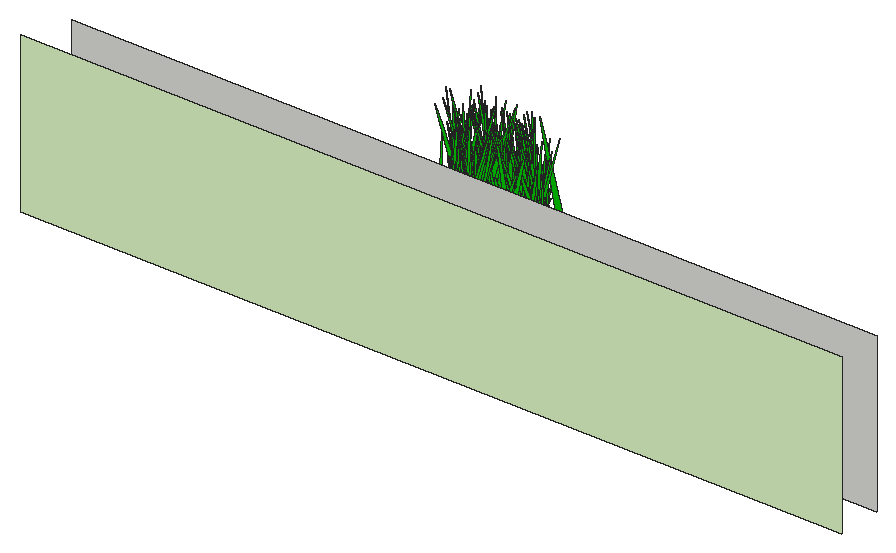
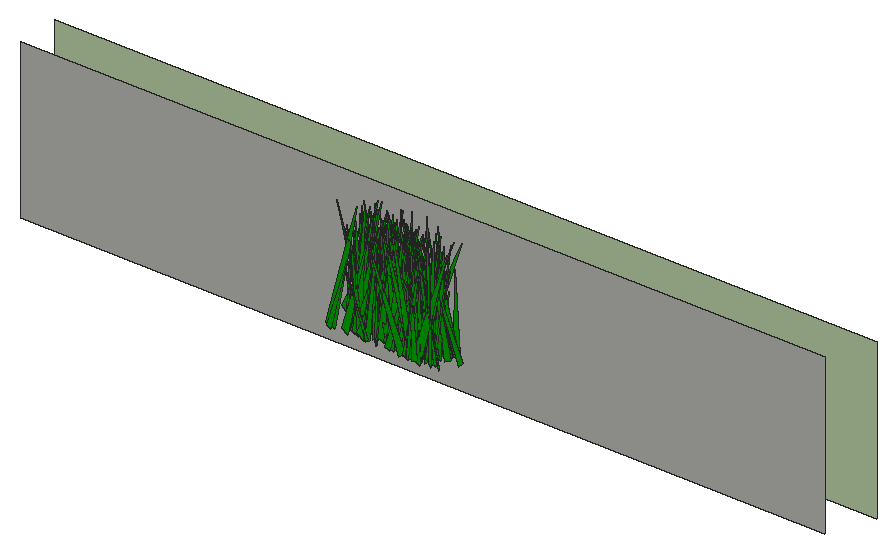
# SketchUp Ruby script. Lengths in inches.
U = 1.inch
M = Sketchup.active_model
def pt(a) = Geom::Point3d.new(a.map { |v| v * U })
def face(e, loops, mat)
  f = e.add_face(loops[0].map { |a| pt(a) })
  loops[1..].each { |l| e.add_face(l.map { |a| pt(a) }).erase! }
  f.material = f.back_material = mat if mat
  f
end
# faces: each face lists its corners as indices into pts; further lists are holes
def faces(e, pts, list, mat = nil) = list.each { |f| face(e, (f[0].is_a?(Array) ? f : [f]).map { |l| l.map { |i| pts[i] } }, mat) }
# xy, xz, yz: faces in a plane at the given z, y or x. An outline is a flat list of corners, or four numbers for a rectangle; further outlines are holes
def ring(l) = l.size == 4 ? [[l[0], l[1]], [l[2], l[1]], [l[2], l[3]], [l[0], l[3]]] : l.each_slice(2).to_a
def flat(e, list, mat, &to3) = list.each { |f| face(e, (f[0].is_a?(Array) ? f : [f]).map { |l| ring(l).map { |u, v| to3.(u, v) } }, mat) }
def xy(e, z, list, mat = nil) = flat(e, list, mat) { |x, y| [x, y, z] }
def xz(e, y, list, mat = nil) = flat(e, list, mat) { |x, z| [x, y, z] }
def yz(e, x, list, mat = nil) = flat(e, list, mat) { |y, z| [x, y, z] }
def lines(e, pts, list) = list.each { |a, b| e.add_line(pt(pts[a]), pt(pts[b])) }
# prism: a flat outline (further loops are holes) pulled along v
def prism(e, loops, v, mat = nil)
  f = face(e, loops, mat); d = Geom::Vector3d.new(v.map { |x| x * U })
  f.pushpull(f.normal.samedirection?(d) ? d.length : -d.length)
end
def box(e, o, s, mat = nil) = prism(e, [[o, [o[0] + s[0], o[1], o[2]], [o[0] + s[0], o[1] + s[1], o[2]], [o[0], o[1] + s[1], o[2]]]], [0, 0, s[2]], mat)
def at(x, y, z, deg = 0) = Geom::Transformation.translation(pt([x, y, z])) * Geom::Transformation.rotation(ORIGIN, Z_AXIS, deg.degrees)
def axes(o, x, y, z) = Geom::Transformation.new([*x, 0, *y, 0, *z, 0, *pt(o).to_a, 1])
def part(name) = M.definitions.add(name)
# library, detail: a bought-in or finely detailed component or shape, given as its bounding box
def library(name, o, s) = part(name).tap { |d| box(d.entities, o, s) }
def detail(e, o, s) = box(e.add_group.entities, o, s)
def put(e, d, t, mat = nil) = e.add_instance(d, t).tap { |i| i.material = mat if mat }
def group(e, t, mat = nil) = e.add_group.tap { |g| g.transformation = t; g.material = mat if mat }.entities
root = M.entities
M.materials.add("[Color F01]1").color = [229, 255, 204]
M.materials.add("[Color G06]").color = [0, 204, 0]
c1 = part("fur_instance\#9")
p = [[0.8125,0,1.79],[0.67,-0.02,1.48],[0,-0.11,0],[0,0.11,0]]
faces(c1.entities,p,[[0,1,2,3]])
xz(root,2.125,[[0,-6,121.48,17.375]],"[Color F01]1")
xz(root,8.54,[[2.44,-6,121.48,17.375]])
put(root,c1,axes([51.91,18.98,4.28],[-5.43727,-0.1309,1.77708],[-1.14633,0.75939,-1.4087],[0.99043,0.16028,8.12542]),"[Color G06]")
put(root,c1,axes([50.8,16.22,4.28],[1.59166,0.55171,0.19188],[3.87124,-0.22097,1.25545],[-0.82664,0.02745,6.24887]),"[Color G06]")
put(root,c1,axes([50.67,17.92,4.28],[2.66118,-0.06056,1.5398],[-0.73116,-0.37487,1.12897],[-0.84584,0.1335,3.86858]),"[Color G06]")
put(root,c1,axes([52.11,18.91,4.28],[-4.41289,-0.15737,0.71019],[-0.90608,0.58635,2.34948],[0.82368,-0.19812,6.38937]),"[Color G06]")
put(root,c1,axes([50.03,20.49,4.28],[3.21331,-0.02062,0.29283],[-0.07963,-0.42686,-1.50113],[-0.23219,-0.13898,4.56724]),"[Color G06]")
put(root,c1,axes([53.29,20.63,4.28],[-0.32371,-0.80099,1.32155],[-5.37319,-0.00581,-3.34481],[-2.21483,0.13118,7.92139]),"[Color G06]")
put(root,c1,axes([50.27,17.08,4.28],[-0.50903,0.54466,0.68853],[3.72815,0.08745,-1.79039],[1.2527,-0.03895,5.60818]),"[Color G06]")
put(root,c1,axes([48.65,18.15,4.28],[3.59181,0.48472,0.30488],[3.26872,-0.45529,-2.86735],[1.19994,-0.21067,6.89826]),"[Color G06]")
put(root,c1,axes([51.4,20.41,4.28],[-3.58351,-0.18608,3.16742],[-1.99042,0.52471,-1.48906],[1.51995,0.24842,5.51771]),"[Color G06]")
put(root,c1,axes([53.17,19.5,4.28],[-2.59947,0.59847,0.19892],[4.24015,0.35436,1.30133],[-0.67711,-0.07856,7.38549]),"[Color G06]")
put(root,c1,axes([51.89,18.54,4.28],[1.47697,-0.74428,0.0462],[-5.2567,-0.20361,-1.42243],[-0.9254,-0.0313,8.15384]),"[Color G06]")
put(root,c1,axes([52.12,20.3,4.28],[-2.67483,-0.2008,0.45513],[-1.28725,0.36186,1.44134],[0.7137,-0.09992,4.30538]),"[Color G06]")
put(root,c1,axes([50.39,18.45,4.28],[2.14413,0.52359,3.01188],[4.23289,-0.22537,-2.23054],[0.49195,-0.34289,6.06514]),"[Color G06]")
put(root,c1,axes([51.79,19.5625,4.28],[-3.356,-0.37288,1.10105],[-2.37095,0.46935,2.11661],[1.43931,-0.09628,6.05393]),"[Color G06]")
put(root,c1,axes([52.37,16.84,4.28],[1.56901,0.37265,0.88402],[2.38955,-0.23286,1.80258],[-1.33471,0.02117,4.2664]),"[Color G06]")
put(root,c1,axes([51.46,20.07,4.28],[-1.02275,-0.37605,1.39838],[-2.66112,0.17575,1.08178],[1.03265,0.08046,4.17267]),"[Color G06]")
put(root,c1,axes([52.05,16.48,4.28],[3.73089,0.48313,0.10401],[2.99318,-0.45646,3.73766],[-1.74634,0.24981,6.62847]),"[Color G06]")
put(root,c1,axes([50.84,17.53,4.28],[1.44178,-0.46037,0.51457],[-3.24906,-0.18502,1.31972],[0.67931,0.09216,5.21997]),"[Color G06]")
put(root,c1,axes([51.3,20.03,4.28],[4.4532,-0.59952,0.68935],[-4.15792,-0.61906,-1.84914],[-1.18686,-0.08069,9.06462]),"[Color G06]")
put(root,c1,axes([53.47,17.11,4.28],[-4.54302,0.12366,0.66916],[0.73291,0.61451,-1.93068],[0.67062,0.16614,6.64316]),"[Color G06]")
put(root,c1,axes([50.8,17.34,4.28],[2.63054,0.38998,0.98746],[2.84635,-0.33642,-1.67464],[0.3952,-0.17281,5.48849]),"[Color G06]")
put(root,c1,axes([55.2,16.72,4.28],[-0.3206,-0.72645,3.92377],[-5.03987,-0.15016,-4.11338],[-2.93792,0.33686,6.62813]),"[Color G06]")
put(root,c1,axes([51.51,19.54,4.28],[5.2193,-0.28703,1.37107],[-1.85383,-0.73035,-1.80051],[-1.28134,-0.11251,8.18977]),"[Color G06]")
put(root,c1,axes([53.89,18,4.28],[-1.41177,0.69633,0.61405],[4.93285,0.18273,1.52968],[-0.87839,-0.093,7.60345]),"[Color G06]")
put(root,c1,axes([51.71,18.59,4.28],[3.12751,-0.10134,1.06954],[-0.89259,-0.42768,1.17512],[-0.4935,0.13131,4.65273]),"[Color G06]")
put(root,c1,axes([51.93,19.64,4.28],[-0.34521,0.71417,0.85118],[5.04938,0.06277,-1.47542],[1.02858,-0.06844,7.52863]),"[Color G06]")
put(root,c1,axes([51.91,17.48,4.28],[5.4788,-0.35623,0.70633],[-2.08372,-0.6944,-4.12755],[-1.55165,-0.32532,8.03693]),"[Color G06]")
put(root,c1,axes([52.09,16.08,4.28],[-3.28322,0.56965,2.82631],[3.90028,0.52294,-1.98729],[2.24771,-0.07533,7.57675]),"[Color G06]")
put(root,c1,axes([53.39,18.09,4.28],[1.26443,0.71457,1.55863],[5.10243,-0.20135,1.35812],[-1.1454,-0.10814,7.77067]),"[Color G06]")
put(root,c1,axes([53.06,20.23,4.28],[2.01762,0.51142,0.00605],[3.4996,-0.26866,1.86814],[-1.09703,0.08354,5.97064]),"[Color G06]")
put(root,c1,axes([53.86,16.875,4.28],[-2.81215,0.18439,1.24159],[1.54852,0.36006,1.69194],[0.2015,-0.19378,4.32525]),"[Color G06]")
put(root,c1,axes([52.39,19.39,4.28],[5.28794,0.45044,0.30203],[2.73932,-0.65163,4.5076],[-1.7237,0.34626,8.09011]),"[Color G06]")
put(root,c1,axes([53.04,20.05,4.28],[-1.73279,-0.44896,0.00822],[-3.13171,0.23524,1.26378],[0.74712,-0.05522,5.31643]),"[Color G06]")
put(root,c1,axes([56.03,17.67,4.28],[-4.70247,0.53813,0.21183],[3.67167,0.61341,3.06077],[-1.19634,-0.23262,8.56112]),"[Color G06]")
put(root,c1,axes([52.2,17.94,4.28],[-0.36312,-0.73049,0.03256],[-5.06328,0.04972,2.01132],[1.34399,-0.01005,7.58611]),"[Color G06]")
put(root,c1,axes([53.14,19.85,4.28],[2.57444,0.09347,1.0726],[0.37331,-0.35287,1.53085],[-0.90827,0.11989,3.66944]),"[Color G06]")
put(root,c1,axes([51.55,17.57,4.28],[4.954,0.01736,0.01736],[0.11791,-0.67006,1.80205],[-0.04155,0.16804,7.18388]),"[Color G06]")
put(root,c1,axes([53.58,18.73,4.28],[-2.17917,0.34186,0.81991],[2.32851,0.31287,-1.1613],[0.9429,0.01744,4.76276]),"[Color G06]")
put(root,c1,axes([51.83,17.94,4.28],[2.92636,-0.57671,1.37096],[-4.19516,-0.37292,1.98178],[0.58866,0.20931,7.30812]),"[Color G06]")
put(root,c1,axes([53.86,19.83,4.28],[0.93646,-0.35885,0.31759],[-2.46765,-0.13365,-1.09467],[-0.76036,-0.0082,3.94375]),"[Color G06]")
put(root,c1,axes([54.26,15.89,4.28],[-3.0515,0.17993,1.51687],[1.52303,0.42177,1.09675],[0.61266,-0.15232,4.82866]),"[Color G06]")
put(root,c1,axes([53.98,16.67,4.28],[-2.96455,0.01566,1.45683],[-0.26452,0.40381,-1.70114],[0.94487,0.16219,4.09459]),"[Color G06]")
put(root,c1,axes([53.41,17.24,4.28],[-2.20301,-0.3923,0.30621],[-2.46722,0.28556,2.37694],[1.36733,-0.11681,4.78234]),"[Color G06]")
put(root,c1,axes([52.2,19.61,4.28],[2.68315,-0.56541,1.54609],[-4.15271,-0.33867,1.87057],[0.51547,0.21471,7.02186]),"[Color G06]")
put(root,c1,axes([54.77,17.11,4.28],[-3.65389,0.39957,2.10603],[3.14363,0.50252,1.23084],[0.56016,-0.21377,6.82994]),"[Color G06]")
put(root,c1,axes([53.4375,20.73,4.28],[-1.09405,-0.45265,0.62127],[-3.12842,0.1626,1.30294],[0.96057,0.01401,4.95104]),"[Color G06]")
put(root,c1,axes([54.01,16.18,4.28],[-3.79355,0.174,2.16516],[1.06017,0.56495,-1.06638],[1.59116,0.03843,5.87255]),"[Color G06]")
put(root,c1,axes([55.3,20.36,4.28],[0.09839,-0.76811,0.41834],[-5.27928,-0.02442,-2.37631],[-1.59654,0.0334,7.88352]),"[Color G06]")
put(root,c1,axes([54.09,17.07,4.28],[-2.01588,0.37847,0.07105],[2.59123,0.27075,-1.45532],[0.80893,0.07587,4.83886]),"[Color G06]")
put(root,c1,axes([54.8125,20.64,4.28],[1.79807,-0.46544,1.83512],[-3.12533,-0.29835,-1.85243],[-1.69731,0.0563,5.35503]),"[Color G06]")
put(root,c1,axes([55.7,20.13,4.28],[-4.8184,-0.1577,1.09211],[-1.30772,0.63828,-2.30012],[0.32064,0.23332,7.03046]),"[Color G06]")
put(root,c1,axes([54.84,20.6,4.28],[-5.6317,-0.0853,2.59145],[-0.41065,0.81772,1.09845],[1.79219,-0.08067,8.39493]),"[Color G06]")
put(root,c1,axes([56.25,17.3,4.28],[-0.91344,0.56581,1.68311],[3.78284,0.03966,3.05415],[-1.84997,-0.19827,5.41411]),"[Color G06]")
put(root,c1,axes([53.04,16.04,4.28],[5.03717,-0.2836,0.52782],[-1.87621,-0.68318,-2.17154],[-0.86065,-0.1705,7.82309]),"[Color G06]")
put(root,c1,axes([54.01,19.33,4.28],[-2.92682,0.64675,1.27318],[4.37587,0.4246,-2.30737],[1.75749,0.01987,7.86524]),"[Color G06]")
put(root,c1,axes([54.18,16.9,4.28],[-4.87066,0.13601,5.05112],[2.2494,0.73928,2.55826],[2.70436,-0.36995,6.96939]),"[Color G06]")
put(root,c1,axes([54.86,18.23,4.28],[3.21289,-0.35741,2.23312],[-2.45895,-0.49264,-1.15504],[-1.65999,0.03798,6.03315]),"[Color G06]")
put(root,c1,axes([55.24,17.59,4.28],[-4.44876,-0.50622,0.53471],[-3.31452,0.59382,2.98091],[1.52335,-0.18632,8.04742]),"[Color G06]")
put(root,c1,axes([56.57,19.68,4.28],[-4.95682,0.3204,1.78327],[2.56581,0.65591,2.3934],[0.34564,-0.27427,7.80688]),"[Color G06]")
put(root,c1,axes([54.06,18.78,4.28],[5.71057,0.15561,1.7452],[0.49355,-0.73778,3.94943],[-1.53791,0.34103,7.74774]),"[Color G06]")
put(root,c1,axes([56.01,16.83,4.28],[-3.14332,-0.06886,0.79043],[-0.6143,0.42769,-1.17654],[0.38237,0.12102,4.6077]),"[Color G06]")
put(root,c1,axes([54.67,19.4,4.28],[4.9091,-0.22213,1.7695],[-1.06395,-0.66635,-3.01583],[-1.67549,-0.22769,7.09963]),"[Color G06]")
put(root,c1,axes([53.87,17.86,4.28],[0.98414,-0.63505,2.16198],[-4.67123,-0.0845,1.89848],[1.00608,0.22887,6.6998]),"[Color G06]")
put(root,c1,axes([57.23,16.93,4.28],[-0.71373,0.56558,2.16635],[3.82854,-0.01056,3.13415],[-1.97327,-0.22505,5.29731]),"[Color G06]")
put(root,c1,axes([53.07,18.01,4.28],[4.3109,0.57571,0.91743],[4.15372,-0.57961,-1.81566],[0.41065,-0.18096,8.7344]),"[Color G06]")
put(root,c1,axes([56.8125,16.01,4.28],[-5.14763,-0.11078,0.62818],[-0.69238,0.70606,1.62962],[0.57303,-0.14201,7.6121]),"[Color G06]")
put(root,c1,axes([54.51,19.01,4.28],[4.6637,0.04467,1.96815],[0.56634,-0.66207,-1.27146],[-1.23126,-0.13533,6.87]),"[Color G06]")
put(root,c1,axes([54.84,16.01,4.28],[-2.53601,-0.44544,1.887],[-2.94328,0.39463,1.86527],[1.77059,0.018,5.8034]),"[Color G06]")
put(root,c1,axes([55.8,19.72,4.28],[-4.87145,-0.24567,2.22206],[-1.45468,0.70359,1.8125],[1.78837,-0.0969,7.52712]),"[Color G06]")
put(root,c1,axes([54.28,16.97,4.28],[3.75989,-0.18432,0.02514],[-1.26237,-0.50274,-1.6992],[-0.39228,-0.14882,5.70906]),"[Color G06]")
put(root,c1,axes([54.05,20.52,4.28],[3.78708,-0.61294,1.46517],[-4.50316,-0.51295,1.34878],[0.0613,0.18561,8.56597]),"[Color G06]")
put(root,c1,axes([57.54,19.3,4.28],[-0.2302,-0.7663,3.67987],[-5.72631,-0.07844,-2.6766],[-1.86297,0.33579,7.77248]),"[Color G06]")
put(root,c1,axes([57.55,18.17,4.28],[-4.41754,0.41018,1.19465],[3.04744,0.59864,1.55983],[0.06736,-0.18307,7.77723]),"[Color G06]")
put(root,c1,axes([57.73,18.14,4.28],[-2.28217,0.3951,0.98803],[2.74251,0.25301,2.52763],[-0.97151,-0.21392,4.81436]),"[Color G06]")
put(root,c1,axes([54.64,16.04,4.28],[4.80796,0.27285,0.51449],[1.85051,-0.66078,1.62678],[-0.72295,0.1232,7.58565]),"[Color G06]")
put(root,c1,axes([55.62,18.85,4.28],[-2.56409,0.55267,1.28765],[3.73312,0.37715,-1.99047],[1.58564,0.00577,6.76845]),"[Color G06]")
put(root,c1,axes([57,16.68,4.28],[-2.39553,-0.28305,0.99137],[-2.13538,0.31619,-1.15524],[-0.02023,0.142,4.54836]),"[Color G06]")
put(root,c1,axes([56.44,18.59,4.28],[-3.57468,0.37857,0.89322],[2.5316,0.49942,-1.68408],[1.14822,0.07745,6.49389]),"[Color G06]")
put(root,c1,axes([56.22,19.31,4.28],[-3.25199,-0.42833,0.48071],[-2.81575,0.43795,2.27741],[1.26886,-0.12592,6.28583]),"[Color G06]")
put(root,c1,axes([56.7,18.07,4.28],[-5.02578,0.41451,1.36063],[2.66068,0.69831,-2.48577],[1.60806,0.14008,8.36541]),"[Color G06]")
put(root,c1,axes([55.55,18.9,4.28],[5.31584,-0.3496,1.58327],[-2.05145,-0.72768,-3.07238],[-1.78863,-0.20441,8.22934]),"[Color G06]")
put(root,c1,axes([55.73,17.21,4.28],[2.97516,0.3331,0.52522],[2.22924,-0.40884,1.57847],[-0.92733,0.08584,5.47962]),"[Color G06]")
put(root,c1,axes([54.18,16.14,4.28],[4.72016,-0.32932,0.82208],[-2.4235,-0.63512,1.85574],[0.08048,0.18904,7.66695]),"[Color G06]")
put(root,c1,axes([53.94,20.49,4.28],[2.61336,-0.7133,1.78302],[-5.079,-0.2958,3.03462],[1.33898,0.27014,8.03086]),"[Color G06]")
put(root,c1,axes([52.64,16.54,4.28],[3.88839,-0.66133,0.92114],[-4.20681,-0.42029,5.00392],[2.27473,0.35318,7.67952]),"[Color G06]")
put(root,c1,axes([57.01,18.27,4.28],[0.09928,0.6289,0.73743],[4.45999,-0.02615,1.22031],[-0.83184,-0.06513,6.63078]),"[Color G06]")
put(root,c1,axes([56.4,18.125,4.28],[-3.14788,-0.71939,1.72009],[-5.10547,0.46218,1.33437],[1.36872,0.06948,8.93334]),"[Color G06]")
put(root,c1,axes([57.7,20.47,4.28],[-1.20173,-0.48488,0.32642],[-3.34679,0.1517,-1.63607],[-0.96834,0.07743,5.24951]),"[Color G06]")
put(root,c1,axes([56.45,18.53,4.28],[-3.24455,0.24157,1.31211],[1.29837,0.44707,-2.28355],[1.44431,0.14078,5.00039]),"[Color G06]")
put(root,c1,axes([54.61,15.99,4.28],[3.56814,-0.46325,0.26466],[-3.29258,-0.48656,1.32268],[0.476,0.10693,7.16534]),"[Color G06]")
put(root,c1,axes([56.65,18.36,4.28],[4.28936,-0.1549,2.53842],[-0.25097,-0.59001,-3.18872],[-2.01387,-0.2564,5.80399]),"[Color G06]")
put(root,c1,axes([58.7,19.6,4.28],[-2.42071,-0.34779,0.35927],[-2.18179,0.26965,-2.85087],[-1.2321,0.2058,4.34246]),"[Color G06]")
put(root,c1,axes([55.77,16.59,4.28],[2.0153,0.3765,1.5154],[2.88365,-0.2601,-1.14271],[0.04918,-0.17695,4.90408]),"[Color G06]")
put(root,c1,axes([57.52,20.24,4.28],[0.89482,-0.73405,1.78711],[-5.23661,-0.15908,-1.64899],[-1.31072,0.13441,7.80815]),"[Color G06]")
put(root,c1,axes([57,18,4.28],[2.87944,0.06028,2.41609],[0.89575,-0.43448,-1.13929],[-1.41345,-0.15254,4.19998]),"[Color G06]")
put(root,c1,axes([55.72,18.04,4.28],[1.49486,-0.57441,0.15573],[-4.06287,-0.20289,1.14753],[0.68695,0.04998,6.44801]),"[Color G06]")
put(root,c1,axes([56.75,18.97,4.28],[-4.2817,-0.58541,2.60043],[-3.99315,0.6438,1.96254],[2.16944,0.0296,8.74461]),"[Color G06]")
put(root,c1,axes([59.28,18.55,4.28],[-6.16398,0.00446,0.29622],[-0.01792,0.83336,-2.2759],[0.19996,0.21231,8.92709]),"[Color G06]")
put(root,c1,axes([55.78,16.93,4.28],[0.20196,0.67568,1.34421],[4.7415,0.00758,-2.02915],[1.34367,-0.12832,6.95834]),"[Color G06]")
put(root,c1,axes([58.15,19.48,4.28],[-4.96916,-0.37311,0.63335],[-2.44496,0.67085,2.5494],[1.16665,-0.18332,8.0405]),"[Color G06]")
put(root,c1,axes([58.1,16.55,4.28],[-3.33094,0.10151,1.09293],[0.89973,0.45444,1.27666],[0.50511,-0.14009,4.93332]),"[Color G06]")
put(root,c1,axes([59.75,17.29,4.28],[-1.76106,0.73325,1.58639],[4.99783,0.16767,3.4903],[-1.94889,-0.23259,7.51719]),"[Color G06]")
put(root,c1,axes([55.82,17.77,4.28],[0.02607,0.52347,2.26385],[3.70064,0.08253,-2.2873],[1.64064,-0.19446,5.12328]),"[Color G06]")
put(root,c1,axes([56.61,16.125,4.28],[-1.26157,0.51868,2.58255],[3.837,0.2383,-1.31112],[1.44861,-0.1795,5.72193]),"[Color G06]")
put(root,c1,axes([57.54,17.97,4.28],[1.91115,0.38665,0.83998],[2.64993,-0.27777,1.2201],[-0.99089,0.00289,4.88298]),"[Color G06]")
put(root,c1,axes([57.68,18.73,4.28],[-3.11151,-0.45224,0.51795],[-3.0544,0.42745,1.88682],[1.14395,-0.08877,6.44672]),"[Color G06]")
put(root,c1,axes([55.51,16.04,4.28],[4.67702,0.23225,0.60128],[1.71295,-0.62979,-1.81715],[0.04177,-0.17849,7.19422]),"[Color G06]")
put(root,c1,axes([58.64,16.68,4.28],[-0.52684,0.57055,1.22282],[4.03527,0.04041,1.71746],[-1.06157,-0.12954,5.9216]),"[Color G06]")
put(root,c1,axes([59.4375,17.36,4.28],[-4.19523,-0.33988,0.94339],[-2.51196,0.55339,-2.04935],[-0.1711,0.20914,6.95587]),"[Color G06]")
put(root,c1,axes([56.38,15.94,4.28],[4.69206,-0.25919,1.77415],[-2.06215,-0.65357,1.21386],[-0.78195,0.16834,7.4445]),"[Color G06]")
put(root,c1,axes([55.08,17.45,4.28],[3.63127,0.64495,2.15055],[4.69378,-0.40661,-3.69554],[1.19603,-0.36239,7.97377]),"[Color G06]")
put(root,c1,axes([56.2,19.58,4.28],[0.70458,0.81412,1.97938],[5.8353,-0.05186,-2.18973],[1.33732,-0.20266,8.51186]),"[Color G06]")
put(root,c1,axes([56.64,19.93,4.28],[-0.72254,-0.69652,2.04973],[-4.94896,0.14983,1.95188],[1.52905,0.15581,7.28607]),"[Color G06]")
put(root,c1,axes([57.56,18.86,4.28],[2.95462,-0.61198,0.5839],[-4.26992,-0.41389,-1.56813],[-1.08657,-0.03764,7.75007]),"[Color G06]")
put(root,c1,axes([55.51,20.54,4.28],[3.63201,-0.5608,0.16417],[-3.79812,-0.47116,2.81005],[1.32659,0.18642,7.59589]),"[Color G06]")
put(root,c1,axes([57.04,18.49,4.28],[0.96081,-0.78066,1.91846],[-5.66561,-0.09902,1.70963],[0.94316,0.20046,8.31548]),"[Color G06]")
put(root,c1,axes([59.49,20.31,4.28],[-5.21835,0.0177,1.63396],[-0.14397,0.7214,-1.92453],[1.09115,0.17981,7.56041]),"[Color G06]")
put(root,c1,axes([60.48,17.36,4.28],[-1.76784,0.57266,1.28932],[3.92784,0.17988,2.85242],[-1.47686,-0.20709,6.0429]),"[Color G06]")
put(root,c1,axes([59.72,16.93,4.28],[-2.41599,0.39074,1.41292],[2.94773,0.30452,1.58494],[-0.23753,-0.19532,5.29768]),"[Color G06]")
put(root,c1,axes([59.74,19.23,4.28],[1.52959,0.68165,3.45387],[5.03204,-0.302,1.869],[-1.97854,-0.24111,7.42359]),"[Color G06]")
put(root,c1,axes([58.77,18.43,4.28],[-3.12089,-0.21213,1.44841],[-1.33071,0.4531,1.21818],[1.21756,-0.04852,5.04398]),"[Color G06]")
put(root,c1,axes([59.61,19.3,4.28],[-0.63491,0.58858,0.91286],[4.20465,0.07198,1.20142],[-0.71378,-0.09956,6.26518]),"[Color G06]")
put(root,c1,axes([62.25,18.44,4.28],[-3.78619,0.6952,0.26747],[4.53583,0.46669,4.07886],[-2.07688,-0.24814,8.42047]),"[Color G06]")
put(root,c1,axes([60.36,18.36,4.28],[-5.22329,0.32936,0.9818],[2.26179,0.73058,-1.27526],[0.94575,0.0718,8.47217]),"[Color G06]")
put(root,c1,axes([59.44,17.84,4.28],[-4.03787,-0.59657,0.40051],[-4.00136,0.54299,2.79815],[1.53731,-0.15362,8.33506]),"[Color G06]")
put(root,c1,axes([58.2,16.96,4.28],[2.92501,-0.11015,0.95],[-0.99431,-0.36461,1.98179],[-0.19851,0.20317,4.07157]),"[Color G06]")
put(root,c1,axes([59.71,18,4.28],[-5.12636,-0.18079,2.7137],[-0.9747,0.7522,1.64386],[2.00691,-0.09649,7.73012]),"[Color G06]")
put(root,c1,axes([59.55,20.3125,4.28],[3.91424,-0.20084,1.92032],[-0.90759,-0.54907,-2.46429],[-1.70337,-0.16895,5.72579]),"[Color G06]")
put(root,c1,axes([61.87,20.2,4.28],[-1.1646,-0.65959,1.03144],[-4.38717,0.10816,-3.11985],[-1.89808,0.15471,6.57826]),"[Color G06]")
put(root,c1,axes([58.59,19.2,4.28],[0.59172,-0.44126,1.11561],[-3.08984,-0.0434,1.6886],[1.01156,0.12553,4.5053]),"[Color G06]")
put(root,c1,axes([58.21,16.19,4.28],[4.97631,-0.12097,1.28887],[-1.09785,-0.66386,2.31057],[-0.53944,0.23511,7.18737]),"[Color G06]")
put(root,c1,axes([58.26,19.4,4.28],[2.1079,-0.59543,0.54371],[-4.22476,-0.27924,1.45668],[0.71888,0.10486,6.96643]),"[Color G06]")
put(root,c1,axes([61.17,17.49,4.28],[-1.55697,0.45986,0.0109],[3.21633,0.2115,1.20905],[-0.72849,-0.04906,5.31471]),"[Color G06]")
put(root,c1,axes([60.46,18.14,4.28],[-4.08408,0.36135,0.62577],[2.28165,0.54208,-2.69533],[1.29784,0.18411,6.70769]),"[Color G06]")
put(root,c1,axes([60.07,18.28,4.28],[3.04426,-0.74568,0.00316],[-5.14747,-0.40872,-2.49001],[-1.44886,-0.11469,8.85306]),"[Color G06]")
put(root,c1,axes([60.27,18.78,4.28],[4.23484,0.13131,3.01099],[0.2538,-0.62884,2.35304],[-2.2093,0.17946,6.04184]),"[Color G06]")
put(root,c1,axes([59.69,18.9,4.28],[3.62888,-0.38197,0.78484],[-2.50456,-0.49916,-2.03908],[-1.22723,-0.11077,6.48214]),"[Color G06]")
put(root,c1,axes([60.6,20.43,4.28],[-3.34402,-0.49695,0.8674],[-3.47918,0.47298,1.16723],[0.96554,-0.01679,7.21009]),"[Color G06]")
put(root,c1,axes([58.19,16.79,4.28],[2.34843,-0.49553,0.30743],[-3.37298,-0.29882,2.22483],[1.1371,0.137,5.96462]),"[Color G06]")
put(root,c1,axes([62.8,17.1,4.28],[-3.86068,-0.53857,0.11618],[-3.68701,0.50915,-2.54587],[-1.15264,0.17523,7.7545]),"[Color G06]")
put(root,c1,axes([59.21,19.09,4.28],[3.80862,0.02919,0.7854],[0.08866,-0.52345,1.27418],[-0.55866,0.11591,5.55664]),"[Color G06]")
put(root,c1,axes([61.8,16.09,4.28],[-2.29533,0.68011,2.59999],[5.13997,0.26706,2.11098],[-0.62799,-0.29995,7.77479]),"[Color G06]")
put(root,c1,axes([59.59,17.74,4.28],[-0.40796,-0.39277,1.49778],[-2.8176,0.09767,1.22783],[0.99951,0.11501,4.07257]),"[Color G06]")
put(root,c1,axes([59.62,19.18,4.28],[-0.27939,0.43211,0.42331],[2.96789,0.04892,-1.3611],[0.93509,-0.02616,4.44651]),"[Color G06]")
put(root,c1,axes([60.25,19.625,4.28],[-1.38892,-0.39022,0.49967],[-2.6951,0.1991,1.12776],[0.82399,-0.00652,4.53091]),"[Color G06]")
put(root,c1,axes([61.65,19.71,4.28],[-0.74313,0.48451,0.56234],[3.35544,0.08391,1.59939],[-0.97728,-0.08031,5.06384]),"[Color G06]")
put(root,c1,axes([61.42,20.11,4.28],[-4.79379,0.00407,1.8367],[-0.25463,0.67165,-1.65563],[1.2026,0.15845,6.97088]),"[Color G06]")
put(root,c1,axes([60.88,17.4,4.28],[4.19545,0.24553,2.8022],[1.20742,-0.62969,2.30011],[-2.27109,0.11881,6.39945]),"[Color G06]")
put(root,c1,axes([59.7,19.11,4.28],[3.19178,-0.00769,0.55967],[-0.14276,-0.43512,1.13201],[-0.35055,0.1072,4.63482]),"[Color G06]")
put(root,c1,axes([62.47,19.5,4.28],[-4.23753,-0.07616,0.20891],[-0.55952,0.55012,-2.31439],[-0.06884,0.2166,5.95152]),"[Color G06]")
put(root,c1,axes([62.8,19.96,4.28],[-3.01273,0.38978,1.047],[2.82904,0.37319,2.22418],[-0.54808,-0.21625,5.72541]),"[Color G06]")
put(root,c1,axes([62.19,18.18,4.28],[-4.87062,-0.21905,2.30699],[-1.93337,0.67547,-1.75008],[1.05468,0.22663,7.44582]),"[Color G06]")
put(root,c1,axes([62.85,19.95,4.28],[-0.88219,-0.79122,0.5745],[-5.49112,0.10439,-2.31909],[-1.47983,0.08431,8.26286]),"[Color G06]")
put(root,c1,axes([62.3,18.01,4.28],[-2.97311,-0.52589,2.46958],[-4.1026,0.40247,-1.18728],[0.34914,0.25098,7.07854]),"[Color G06]")
put(root,c1,axes([61.09,18.7,4.28],[-1.14665,-0.76916,0.94314],[-5.46083,0.17246,1.32624],[1.00106,0.05974,8.31498]),"[Color G06]")
put(root,c1,axes([64.27,16.7,4.28],[-3.36704,0.556,0.56613],[3.70439,0.40607,3.40018],[-1.5228,-0.24154,7.01959]),"[Color G06]")
put(root,c1,axes([64.75,17.44,4.28],[-2.7423,0.70777,1.27761],[4.75239,0.29631,3.92937],[-1.97663,-0.26952,7.67483]),"[Color G06]")
put(root,c1,axes([61.7,16.83,4.28],[-4.13962,-0.02647,3.24829],[0.72845,0.59596,2.63163],[2.05646,-0.26439,5.60657]),"[Color G06]")
put(root,c1,axes([62.43,18.26,4.28],[-5.19693,-0.07805,2.56229],[-0.34586,0.7588,1.08839],[1.76998,-0.0809,7.73593]),"[Color G06]")
put(root,c1,axes([60.35,15.92,4.28],[0.99414,0.66846,1.63414],[4.72791,-0.08726,-2.32435],[1.34978,-0.18668,6.93798]),"[Color G06]")
put(root,c1,axes([60.12,17.57,4.28],[0.70211,0.56718,0.09915],[3.67577,-0.08443,-2.65817],[1.74267,-0.05042,5.56685]),"[Color G06]")
put(root,c1,axes([63.36,19.51,4.28],[-3.52071,-0.57985,2.46076],[-4.47208,0.45952,-1.85372],[0.04712,0.28737,7.9294]),"[Color G06]")
put(root,c1,axes([61.04,16.32,4.28],[5.2548,-0.07745,1.86531],[-0.35982,-0.74576,-1.29291],[-1.31783,-0.10522,7.79088]),"[Color G06]")
put(root,c1,axes([60.7,20.48,4.28],[1.99638,0.27508,0.62814],[1.92889,-0.23629,-1.80696],[0.58946,-0.15843,3.78551]),"[Color G06]")
put(root,c1,axes([63.21,17.47,4.28],[2.19271,-0.74854,0.82049],[-4.88636,-0.3105,-3.37182],[-2.2891,-0.05421,7.98351]),"[Color G06]")
put(root,c1,axes([62.4,20.08,4.28],[2.72299,-0.77668,1.07193],[-5.39405,-0.39265,-2.07478],[-1.56248,0.00198,9.03076]),"[Color G06]")
put(root,c1,axes([61.23,16.95,4.28],[5.72063,0.01587,1.97077],[-0.29691,-0.77957,2.6463],[-1.28978,0.24985,8.13184]),"[Color G06]")
put(root,c1,axes([61.35,19.2,4.28],[1.32667,-0.35602,0.17914],[-2.47684,-0.17443,1.15143],[0.63097,0.06387,4.14324]),"[Color G06]")
put(root,c1,axes([62.4375,18.85,4.28],[-4.58423,-0.28528,4.18963],[-2.73133,0.69611,-1.23077],[2.14083,0.27725,7.40112]),"[Color G06]")
put(root,c1,axes([62.43,19.93,4.28],[3.17751,0.00474,2.0851],[-0.36394,-0.46424,1.36003],[-1.34723,0.13658,4.5504]),"[Color G06]")
put(root,c1,axes([63.94,17.375,4.28],[-0.3468,-0.48671,0.92706],[-3.28071,0.01113,-2.06993],[-1.34321,0.09847,4.8163]),"[Color G06]")
put(root,c1,axes([63.4,16.33,4.28],[0.2642,0.51374,0.39882],[3.55442,-0.04551,1.47467],[-1.00511,-0.0259,5.31976]),"[Color G06]")
put(root,c1,axes([61.98,20.05,4.28],[1.87648,-0.45806,2.61745],[-3.71971,-0.24139,1.10393],[-0.14523,0.26427,5.54523]),"[Color G06]")
put(root,c1,axes([64.13,20.22,4.28],[0.42786,-0.64547,1.20064],[-4.30678,-0.09883,-2.67513],[-1.87695,0.07963,6.41193]),"[Color G06]")
put(root,c1,axes([61.11,16.53,4.28],[4.10799,-0.34305,1.14453],[-2.5729,-0.55688,1.45354],[-0.13727,0.17155,7.0073]),"[Color G06]")
put(root,c1,axes([64.21,19.3,4.28],[-2.48764,-0.30258,1.19033],[-2.27291,0.29056,-2.12583],[-0.42019,0.21964,4.45212]),"[Color G06]")
put(root,c1,axes([63.6,18.29,4.28],[0.97681,-0.65939,2.14196],[-4.76745,-0.1793,-1.48425],[-1.29823,0.16231,7.06222]),"[Color G06]")
put(root,c1,axes([64.6,19.63,4.28],[-6.02298,0.11871,1.73042],[1.16513,0.81058,2.67103],[0.84122,-0.27278,8.69001]),"[Color G06]")
put(root,c1,axes([61.95,16.68,4.28],[1.47153,-0.52893,1.0028],[-3.82555,-0.18896,1.09009],[0.45043,0.1231,5.98221]),"[Color G06]")
put(root,c1,axes([61.875,18.4,4.28],[0.27472,-0.42718,0.26623],[-2.84077,-0.02597,1.76032],[1.16037,0.03755,4.24652]),"[Color G06]")
put(root,c1,axes([62.75,17.61,4.28],[-4.55342,0.52537,0.45512],[2.91211,0.52998,-5.19788],[2.4097,0.35226,7.14159]),"[Color G06]")
put(root,c1,axes([62.6875,18.81,4.28],[2.76485,0.17715,0.46589],[1.09823,-0.36958,1.58508],[-0.71061,0.11808,4.26242]),"[Color G06]")
put(root,c1,axes([62.3,19.19,4.28],[-1.8631,-0.74113,0.19962],[-4.98576,0.25041,2.85695],[1.84599,-0.07167,7.91768]),"[Color G06]")
put(root,c1,axes([64.52,17.6,4.28],[0.99905,-0.82082,0.21422],[-5.58086,-0.13847,-2.81026],[-1.8771,-0.02518,8.4693]),"[Color G06]")
put(root,c1,axes([65.07,16.93,4.28],[-4.17107,0.5412,2.49579],[4.22391,0.52634,2.65717],[-0.10056,-0.33984,8.09003]),"[Color G06]")
put(root,c1,axes([64.67,16.96,4.28],[0.72682,-0.705,1.77486],[-4.88656,-0.14945,-2.34965],[-1.75841,0.12393,7.26321]),"[Color G06]")
put(root,c1,axes([62.125,19.24,4.28],[3.7312,-0.34943,1.30516],[-2.64761,-0.50436,1.39562],[-0.17878,0.17653,6.57087]),"[Color G06]")
put(root,c1,axes([62.42,19.22,4.28],[3.20878,-0.03067,0.3145],[-0.14105,-0.42515,-1.54862],[-0.26976,-0.14256,4.55072]),"[Color G06]")
put(root,c1,axes([62.92,19.26,4.28],[4.88474,0.30601,1.17491],[1.72637,-0.64594,3.29378],[-1.56634,0.24239,7.29432]),"[Color G06]")
put(root,c1,axes([62.69,19.93,4.28],[2.44126,0.18274,0.9366],[1.44166,-0.32576,-1.09236],[-0.17817,-0.13193,3.99445]),"[Color G06]")
put(root,c1,axes([65.75,17.49,4.28],[-4.90585,0.47903,2.05794],[3.69974,0.62679,2.94087],[-0.0928,-0.33465,8.45409]),"[Color G06]")
put(root,c1,axes([62.67,18.69,4.28],[3.79636,0.08693,1.5617],[1.08379,-0.45859,-2.95264],[-0.55305,-0.30195,4.93393]),"[Color G06]")
put(root,c1,axes([63.44,16.46,4.28],[-1.78933,0.46032,1.41665],[3.15172,0.2793,-1.53306],[1.3646,-0.04148,5.3984]),"[Color G06]")
put(root,c1,axes([63.17,16.52,4.28],[-1.46364,-0.52556,2.31],[-3.69474,0.26772,1.76779],[1.71543,0.1282,5.77845]),"[Color G06]")
put(root,c1,axes([64.24,16.96,4.28],[3.1486,0.54504,1.50673],[3.74943,-0.46094,1.65255],[-1.49516,-0.00813,7.31708]),"[Color G06]")
put(root,c1,axes([67.29,16.24,4.28],[-3.01706,-0.69436,0.82897],[-4.5539,0.3424,-4.07616],[-2.08917,0.25641,7.6879]),"[Color G06]")
put(root,c1,axes([65.61,17.35,4.28],[-0.48255,-0.73205,2.46523],[-5.34408,0.0073,-2.08763],[-1.31185,0.23954,7.59756]),"[Color G06]")
put(root,c1,axes([64.58,19.11,4.28],[1.01609,0.42923,0.47719],[2.99461,-0.1482,1.06964],[-0.78051,-0.0098,4.72512]),"[Color G06]")
put(root,c1,axes([65.82,16.92,4.28],[-2.93721,-0.50713,1.71879],[-3.80424,0.37484,-1.81689],[-0.27622,0.23015,6.74636]),"[Color G06]")
put(root,c1,axes([62.66,17.57,4.28],[2.08105,0.34184,0.2795],[2.23888,-0.24939,-2.19864],[1.01575,-0.15066,4.27355]),"[Color G06]")
put(root,c1,axes([64.01,17.08,4.28],[4.24311,0.05678,2.05878],[-0.29954,-0.55089,3.12444],[-1.40485,0.28896,5.552]),"[Color G06]")
put(root,c1,axes([66.29,20.2,4.28],[-0.84459,-0.85795,0.75498],[-5.97841,0.09595,-2.41385],[-1.53902,0.09811,8.96241]),"[Color G06]")
put(root,c1,axes([62.65,18.14,4.28],[5.37009,-0.27088,1.02743],[-2.05622,-0.72184,2.14492],[-0.134,0.22111,8.26104]),"[Color G06]")
put(root,c1,axes([65.56,16.92,4.28],[0.88568,-0.44671,0.53264],[-2.93159,-0.13306,-1.93088],[-1.33985,-0.00415,4.57685]),"[Color G06]")
put(root,c1,axes([64.87,17.25,4.28],[-3.27488,0.35861,1.51373],[2.30601,0.47522,-1.78886],[1.52372,0.05155,5.96068]),"[Color G06]")
put(root,c1,axes([66.21,20.62,4.28],[-1.42611,-0.44964,0.66051],[-3.15404,0.17433,-1.57859],[-0.80297,0.11381,5.02755]),"[Color G06]")
